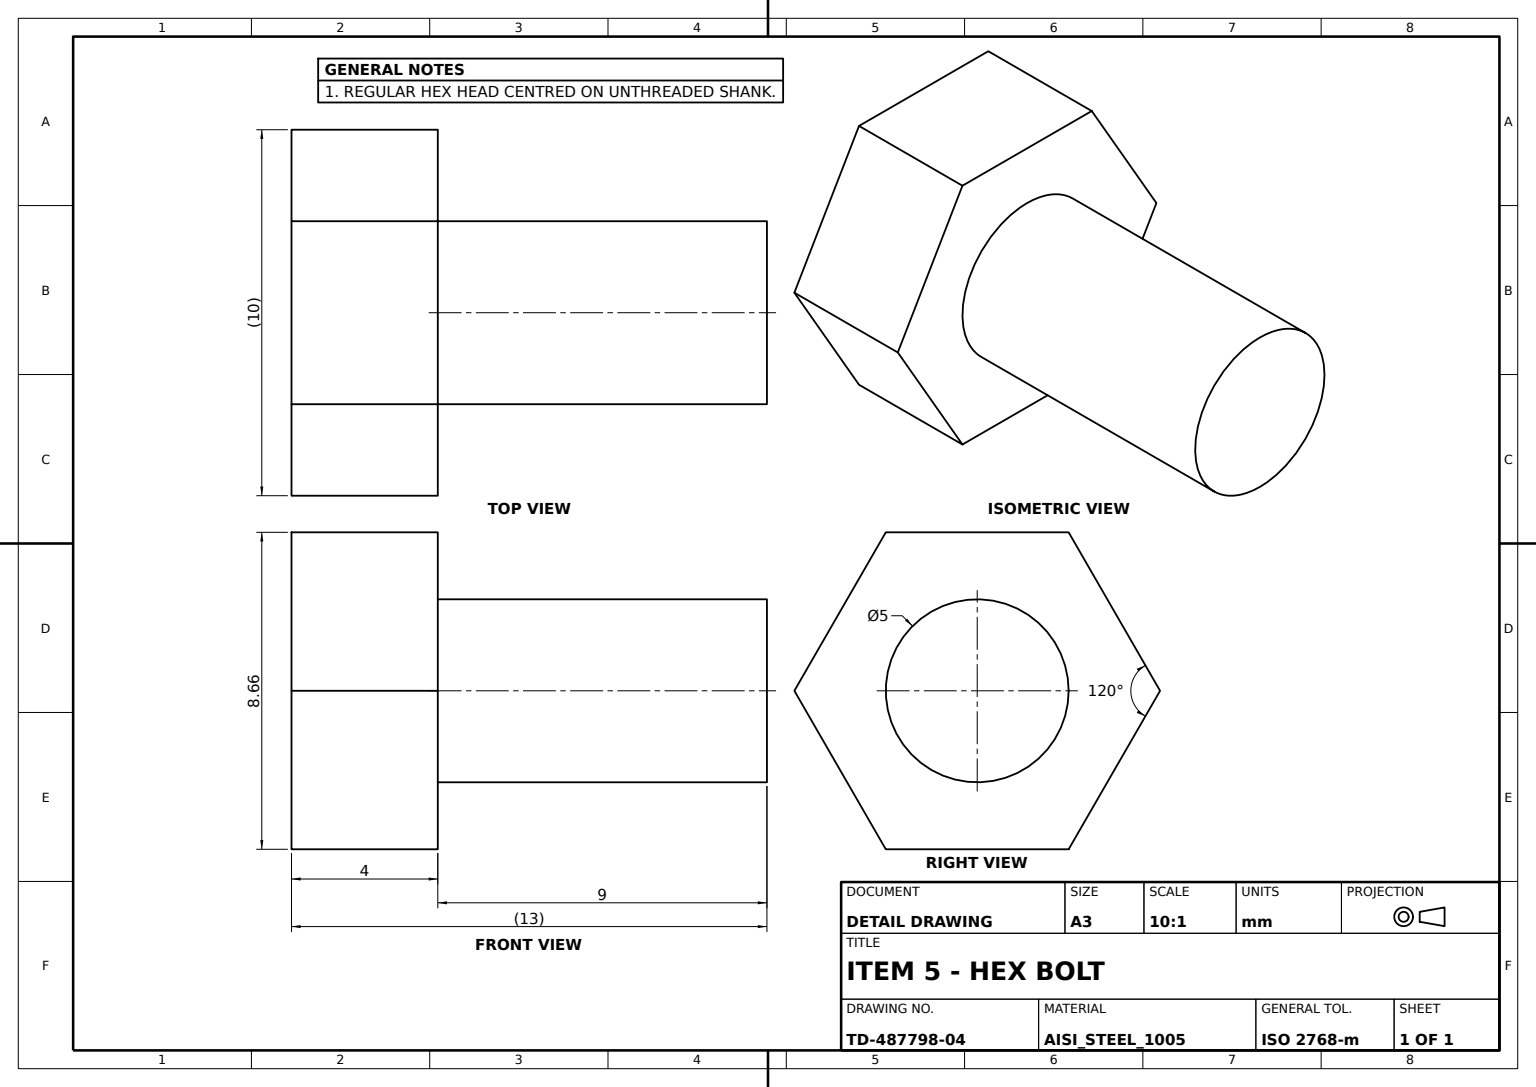
ISO-10303-21;
HEADER;
FILE_DESCRIPTION((''),'2;1');
FILE_NAME('','',(''),(''),'','','');
FILE_SCHEMA(('AUTOMOTIVE_DESIGN'));
ENDSEC;
DATA;
#1=APPLICATION_CONTEXT('');
#2=PRODUCT_CONTEXT('',#1,'mechanical');
#3=PRODUCT('','','',(#2));
#4=PRODUCT_DEFINITION_FORMATION('','',#3);
#5=PRODUCT_DEFINITION_CONTEXT('',#1,'design');
#6=PRODUCT_DEFINITION('','',#4,#5);
#7=PRODUCT_DEFINITION_SHAPE('','',#6);
#8=(LENGTH_UNIT()NAMED_UNIT(*)SI_UNIT(.MILLI.,.METRE.));
#9=(NAMED_UNIT(*)PLANE_ANGLE_UNIT()SI_UNIT($,.RADIAN.));
#10=(NAMED_UNIT(*)SI_UNIT($,.STERADIAN.)SOLID_ANGLE_UNIT());
#11=UNCERTAINTY_MEASURE_WITH_UNIT(LENGTH_MEASURE(0.005),#8,'distance_accuracy_value','');
#12=(GEOMETRIC_REPRESENTATION_CONTEXT(3)GLOBAL_UNCERTAINTY_ASSIGNED_CONTEXT((#11))GLOBAL_UNIT_ASSIGNED_CONTEXT((#8,#9,#10))REPRESENTATION_CONTEXT('',''));
#13=CARTESIAN_POINT('',(2.5,0.,9.));
#14=VERTEX_POINT('',#13);
#15=CARTESIAN_POINT('',(0.,0.,9.));
#16=DIRECTION('',(0.,0.,-1.));
#17=DIRECTION('',(1.,0.,0.));
#18=AXIS2_PLACEMENT_3D('',#15,#16,#17);
#19=CIRCLE('',#18,2.5);
#20=EDGE_CURVE('',#14,#14,#19,.T.);
#21=ORIENTED_EDGE('',*,*,#20,.F.);
#22=EDGE_LOOP('',(#21));
#23=FACE_BOUND('',#22,.T.);
#24=CARTESIAN_POINT('',(-2.5,4.330127,9.));
#25=VERTEX_POINT('',#24);
#26=CARTESIAN_POINT('',(2.5,4.330127,9.));
#27=VERTEX_POINT('',#26);
#28=VECTOR('',#17,1000.);
#29=LINE('',#24,#28);
#30=EDGE_CURVE('',#25,#27,#29,.T.);
#31=ORIENTED_EDGE('',*,*,#30,.T.);
#32=CARTESIAN_POINT('',(5.,0.,9.));
#33=VERTEX_POINT('',#32);
#34=DIRECTION('',(0.5,-0.866025404,0.));
#35=VECTOR('',#34,1000.);
#36=LINE('',#26,#35);
#37=EDGE_CURVE('',#27,#33,#36,.T.);
#38=ORIENTED_EDGE('',*,*,#37,.T.);
#39=CARTESIAN_POINT('',(2.5,-4.330127,9.));
#40=VERTEX_POINT('',#39);
#41=DIRECTION('',(-0.5,-0.866025404,0.));
#42=VECTOR('',#41,1000.);
#43=LINE('',#32,#42);
#44=EDGE_CURVE('',#33,#40,#43,.T.);
#45=ORIENTED_EDGE('',*,*,#44,.T.);
#46=CARTESIAN_POINT('',(-2.5,-4.330127,9.));
#47=VERTEX_POINT('',#46);
#48=DIRECTION('',(-1.,0.,0.));
#49=VECTOR('',#48,1000.);
#50=LINE('',#39,#49);
#51=EDGE_CURVE('',#40,#47,#50,.T.);
#52=ORIENTED_EDGE('',*,*,#51,.T.);
#53=CARTESIAN_POINT('',(-5.,0.,9.));
#54=VERTEX_POINT('',#53);
#55=DIRECTION('',(-0.5,0.866025404,0.));
#56=VECTOR('',#55,1000.);
#57=LINE('',#46,#56);
#58=EDGE_CURVE('',#47,#54,#57,.T.);
#59=ORIENTED_EDGE('',*,*,#58,.T.);
#60=DIRECTION('',(0.5,0.866025404,0.));
#61=VECTOR('',#60,1000.);
#62=LINE('',#53,#61);
#63=EDGE_CURVE('',#54,#25,#62,.T.);
#64=ORIENTED_EDGE('',*,*,#63,.T.);
#65=EDGE_LOOP('',(#31,#38,#45,#52,#59,#64));
#66=FACE_BOUND('',#65,.T.);
#67=AXIS2_PLACEMENT_3D('',#15,#16,#48);
#68=PLANE('',#67);
#69=ADVANCED_FACE('',(#23,#66),#68,.T.);
#70=CARTESIAN_POINT('',(-5.,0.,13.));
#71=VERTEX_POINT('',#70);
#72=VECTOR('',#16,1000.);
#73=LINE('',#70,#72);
#74=EDGE_CURVE('',#71,#54,#73,.T.);
#75=ORIENTED_EDGE('',*,*,#74,.T.);
#76=ORIENTED_EDGE('',*,*,#58,.F.);
#77=CARTESIAN_POINT('',(-2.5,-4.330127,13.));
#78=VERTEX_POINT('',#77);
#79=LINE('',#77,#72);
#80=EDGE_CURVE('',#78,#47,#79,.T.);
#81=ORIENTED_EDGE('',*,*,#80,.F.);
#82=LINE('',#77,#56);
#83=EDGE_CURVE('',#78,#71,#82,.T.);
#84=ORIENTED_EDGE('',*,*,#83,.T.);
#85=EDGE_LOOP('',(#75,#76,#81,#84));
#86=FACE_BOUND('',#85,.T.);
#87=DIRECTION('',(-0.866025404,-0.5,0.));
#88=AXIS2_PLACEMENT_3D('',#77,#87,#34);
#89=PLANE('',#88);
#90=ADVANCED_FACE('',(#86),#89,.T.);
#91=CARTESIAN_POINT('',(2.5,0.,0.));
#92=VERTEX_POINT('',#91);
#93=CARTESIAN_POINT('',(0.,0.,0.));
#94=AXIS2_PLACEMENT_3D('',#93,#16,#17);
#95=CIRCLE('',#94,2.5);
#96=EDGE_CURVE('',#92,#92,#95,.T.);
#97=ORIENTED_EDGE('',*,*,#96,.T.);
#98=EDGE_LOOP('',(#97));
#99=FACE_BOUND('',#98,.T.);
#100=AXIS2_PLACEMENT_3D('',#93,#16,#48);
#101=PLANE('',#100);
#102=ADVANCED_FACE('',(#99),#101,.T.);
#103=ORIENTED_EDGE('',*,*,#30,.F.);
#104=CARTESIAN_POINT('',(-2.5,4.330127,13.));
#105=VERTEX_POINT('',#104);
#106=LINE('',#104,#72);
#107=EDGE_CURVE('',#105,#25,#106,.T.);
#108=ORIENTED_EDGE('',*,*,#107,.F.);
#109=CARTESIAN_POINT('',(2.5,4.330127,13.));
#110=VERTEX_POINT('',#109);
#111=LINE('',#104,#28);
#112=EDGE_CURVE('',#105,#110,#111,.T.);
#113=ORIENTED_EDGE('',*,*,#112,.T.);
#114=LINE('',#109,#72);
#115=EDGE_CURVE('',#110,#27,#114,.T.);
#116=ORIENTED_EDGE('',*,*,#115,.T.);
#117=EDGE_LOOP('',(#103,#108,#113,#116));
#118=FACE_BOUND('',#117,.T.);
#119=DIRECTION('',(0.,1.,0.));
#120=AXIS2_PLACEMENT_3D('',#104,#119,#48);
#121=PLANE('',#120);
#122=ADVANCED_FACE('',(#118),#121,.T.);
#123=CARTESIAN_POINT('',(5.,0.,13.));
#124=VERTEX_POINT('',#123);
#125=LINE('',#109,#35);
#126=EDGE_CURVE('',#110,#124,#125,.T.);
#127=ORIENTED_EDGE('',*,*,#126,.F.);
#128=ORIENTED_EDGE('',*,*,#112,.F.);
#129=LINE('',#70,#61);
#130=EDGE_CURVE('',#71,#105,#129,.T.);
#131=ORIENTED_EDGE('',*,*,#130,.F.);
#132=ORIENTED_EDGE('',*,*,#83,.F.);
#133=CARTESIAN_POINT('',(2.5,-4.330127,13.));
#134=VERTEX_POINT('',#133);
#135=LINE('',#133,#49);
#136=EDGE_CURVE('',#134,#78,#135,.T.);
#137=ORIENTED_EDGE('',*,*,#136,.F.);
#138=LINE('',#123,#42);
#139=EDGE_CURVE('',#124,#134,#138,.T.);
#140=ORIENTED_EDGE('',*,*,#139,.F.);
#141=EDGE_LOOP('',(#127,#128,#131,#132,#137,#140));
#142=FACE_BOUND('',#141,.T.);
#143=CARTESIAN_POINT('',(0.,0.,13.));
#144=AXIS2_PLACEMENT_3D('',#143,#16,#48);
#145=PLANE('',#144);
#146=ADVANCED_FACE('',(#142),#145,.F.);
#147=LINE('',#123,#72);
#148=EDGE_CURVE('',#124,#33,#147,.T.);
#149=ORIENTED_EDGE('',*,*,#148,.T.);
#150=ORIENTED_EDGE('',*,*,#37,.F.);
#151=ORIENTED_EDGE('',*,*,#115,.F.);
#152=ORIENTED_EDGE('',*,*,#126,.T.);
#153=EDGE_LOOP('',(#149,#150,#151,#152));
#154=FACE_BOUND('',#153,.T.);
#155=DIRECTION('',(0.866025404,0.5,0.));
#156=AXIS2_PLACEMENT_3D('',#109,#155,#55);
#157=PLANE('',#156);
#158=ADVANCED_FACE('',(#154),#157,.T.);
#159=ORIENTED_EDGE('',*,*,#148,.F.);
#160=ORIENTED_EDGE('',*,*,#139,.T.);
#161=LINE('',#133,#72);
#162=EDGE_CURVE('',#134,#40,#161,.T.);
#163=ORIENTED_EDGE('',*,*,#162,.T.);
#164=ORIENTED_EDGE('',*,*,#44,.F.);
#165=EDGE_LOOP('',(#159,#160,#163,#164));
#166=FACE_BOUND('',#165,.T.);
#167=DIRECTION('',(0.866025404,-0.5,0.));
#168=AXIS2_PLACEMENT_3D('',#123,#167,#60);
#169=PLANE('',#168);
#170=ADVANCED_FACE('',(#166),#169,.T.);
#171=ORIENTED_EDGE('',*,*,#80,.T.);
#172=ORIENTED_EDGE('',*,*,#51,.F.);
#173=ORIENTED_EDGE('',*,*,#162,.F.);
#174=ORIENTED_EDGE('',*,*,#136,.T.);
#175=EDGE_LOOP('',(#171,#172,#173,#174));
#176=FACE_BOUND('',#175,.T.);
#177=DIRECTION('',(0.,-1.,0.));
#178=AXIS2_PLACEMENT_3D('',#133,#177,#17);
#179=PLANE('',#178);
#180=ADVANCED_FACE('',(#176),#179,.T.);
#181=ORIENTED_EDGE('',*,*,#63,.F.);
#182=ORIENTED_EDGE('',*,*,#74,.F.);
#183=ORIENTED_EDGE('',*,*,#130,.T.);
#184=ORIENTED_EDGE('',*,*,#107,.T.);
#185=EDGE_LOOP('',(#181,#182,#183,#184));
#186=FACE_BOUND('',#185,.T.);
#187=DIRECTION('',(-0.866025404,0.5,0.));
#188=AXIS2_PLACEMENT_3D('',#70,#187,#41);
#189=PLANE('',#188);
#190=ADVANCED_FACE('',(#186),#189,.T.);
#191=ORIENTED_EDGE('',*,*,#20,.T.);
#192=EDGE_LOOP('',(#191));
#193=FACE_BOUND('',#192,.T.);
#194=ORIENTED_EDGE('',*,*,#96,.F.);
#195=EDGE_LOOP('',(#194));
#196=FACE_BOUND('',#195,.T.);
#197=CYLINDRICAL_SURFACE('',#67,2.5);
#198=ADVANCED_FACE('',(#193,#196),#197,.T.);
#199=CLOSED_SHELL('',(#69,#90,#102,#122,#146,#158,#170,#180,#190,#198));
#200=MANIFOLD_SOLID_BREP('',#199);
#201=ADVANCED_BREP_SHAPE_REPRESENTATION('',(#200),#12);
#202=SHAPE_DEFINITION_REPRESENTATION(#7,#201);
ENDSEC;
END-ISO-10303-21;
